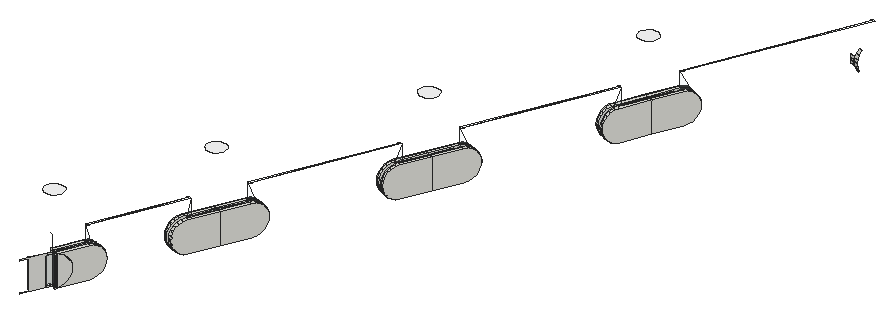
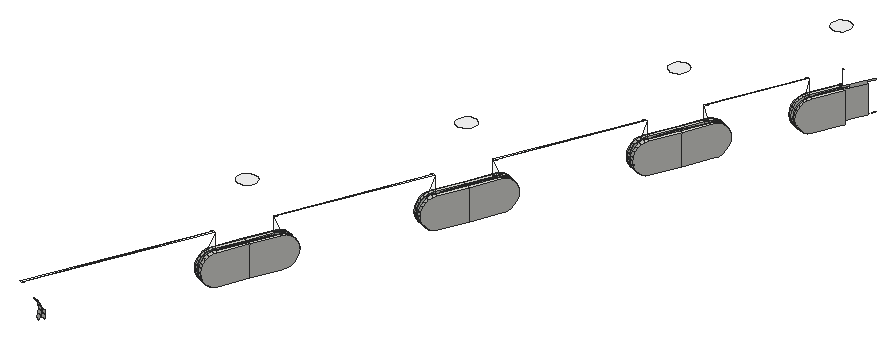
# SketchUp Ruby script. Lengths in inches.
U = 1.inch
M = Sketchup.active_model
def pt(a) = Geom::Point3d.new(a.map { |v| v * U })
def face(e, loops, mat)
  f = e.add_face(loops[0].map { |a| pt(a) })
  loops[1..].each { |l| e.add_face(l.map { |a| pt(a) }).erase! }
  f.material = f.back_material = mat if mat
  f
end
# faces: each face lists its corners as indices into pts; further lists are holes
def faces(e, pts, list, mat = nil) = list.each { |f| face(e, (f[0].is_a?(Array) ? f : [f]).map { |l| l.map { |i| pts[i] } }, mat) }
# xy, xz, yz: faces in a plane at the given z, y or x. An outline is a flat list of corners, or four numbers for a rectangle; further outlines are holes
def ring(l) = l.size == 4 ? [[l[0], l[1]], [l[2], l[1]], [l[2], l[3]], [l[0], l[3]]] : l.each_slice(2).to_a
def flat(e, list, mat, &to3) = list.each { |f| face(e, (f[0].is_a?(Array) ? f : [f]).map { |l| ring(l).map { |u, v| to3.(u, v) } }, mat) }
def xy(e, z, list, mat = nil) = flat(e, list, mat) { |x, y| [x, y, z] }
def xz(e, y, list, mat = nil) = flat(e, list, mat) { |x, z| [x, y, z] }
def yz(e, x, list, mat = nil) = flat(e, list, mat) { |y, z| [x, y, z] }
def lines(e, pts, list) = list.each { |a, b| e.add_line(pt(pts[a]), pt(pts[b])) }
# prism: a flat outline (further loops are holes) pulled along v
def prism(e, loops, v, mat = nil)
  f = face(e, loops, mat); d = Geom::Vector3d.new(v.map { |x| x * U })
  f.pushpull(f.normal.samedirection?(d) ? d.length : -d.length)
end
def box(e, o, s, mat = nil) = prism(e, [[o, [o[0] + s[0], o[1], o[2]], [o[0] + s[0], o[1] + s[1], o[2]], [o[0], o[1] + s[1], o[2]]]], [0, 0, s[2]], mat)
def at(x, y, z, deg = 0) = Geom::Transformation.translation(pt([x, y, z])) * Geom::Transformation.rotation(ORIGIN, Z_AXIS, deg.degrees)
def axes(o, x, y, z) = Geom::Transformation.new([*x, 0, *y, 0, *z, 0, *pt(o).to_a, 1])
def part(name) = M.definitions.add(name)
# library, detail: a bought-in or finely detailed component or shape, given as its bounding box
def library(name, o, s) = part(name).tap { |d| box(d.entities, o, s) }
def detail(e, o, s) = box(e.add_group.entities, o, s)
def put(e, d, t, mat = nil) = e.add_instance(d, t).tap { |i| i.material = mat if mat }
def group(e, t, mat = nil) = e.add_group.tap { |g| g.transformation = t; g.material = mat if mat }.entities
root = M.entities
M.materials.add("Glass_Safety_01").color = [204, 235, 244]
M.materials["Glass_Safety_01"].alpha = 0.1
M.materials.add("[Color_000]").color = [255, 255, 255]
xy(root,351.283,[[844.286,537.43,844.039,537.551,844.043,537.56,844.044,537.562,844.108,537.692,844.355,537.571],[844.362,537.586,844.11,537.696,844.896,539.501,845.148,539.391],[843.931,537.779,843.684,537.9,844.463,539.689,844.715,539.579],[847.571,544.953,847.318,545.063,847.473,545.418,848.104,546.868,848.357,546.758],[847.138,545.142,846.885,545.252,847.671,547.057,847.924,546.947,847.293,545.497],
  [848.357,546.758,848.104,546.868,848.89,548.673,849.143,548.563],[847.924,546.947,847.671,547.057,848.457,548.861,848.71,548.751],[852.79,556.936,852.537,557.046,852.656,557.318,853.323,558.851,853.576,558.741],[852.357,557.125,852.104,557.235,852.89,559.04,853.143,558.93,852.475,557.397],[853.576,558.741,853.323,558.851,854.109,560.656,854.362,560.546],
  [853.143,558.93,852.89,559.04,853.676,560.845,853.929,560.735],[858.192,569.34,857.939,569.45,858.054,569.713,858.726,571.255,858.978,571.145],[857.759,569.529,857.506,569.639,858.292,571.443,858.545,571.333,857.873,569.791],[858.978,571.145,858.726,571.255,859.512,573.06,859.764,572.949],[858.545,571.333,858.292,571.443,859.078,573.248,859.331,573.138]])
xy(root,351.362,[[843.866,537.198,843.689,537.285,843.862,537.638,843.867,537.648,843.929,537.775,844.019,537.735,844.108,537.692,844.044,537.562,844.043,537.56,844.039,537.551],[844.11,537.696,844.019,537.735,843.931,537.779,844.558,539.218,844.738,539.14],[844.019,537.735,843.929,537.775,843.931,537.779],[847.476,545.424,847.295,545.503,847.924,546.947,848.104,546.868],[848.104,546.868,847.924,546.947,848.553,548.39,848.733,548.312],
  [852.695,557.407,852.514,557.486,853.143,558.93,853.323,558.851],[853.323,558.851,853.143,558.93,853.772,560.374,853.952,560.295],[858.097,569.811,857.916,569.89,858.545,571.333,858.726,571.255],[858.726,571.255,858.545,571.333,859.174,572.777,859.354,572.699]],"Glass_Safety_01")
xy(root,353.33,[[844.11,537.696,844.738,539.14,844.558,539.218,843.931,537.779,844.019,537.735],[844.019,537.735,843.931,537.779,843.929,537.775],[847.476,545.424,848.104,546.868,847.924,546.947,847.295,545.503],[848.104,546.868,848.733,548.312,848.553,548.39,847.924,546.947],[852.695,557.407,853.323,558.851,853.143,558.93,852.514,557.486],
  [853.323,558.851,853.952,560.295,853.772,560.374,853.143,558.93],[858.097,569.811,858.726,571.255,858.545,571.333,857.916,569.89],[858.726,571.255,859.354,572.699,859.174,572.777,858.545,571.333]],"Glass_Safety_01")
xy(root,353.409,[[844.286,537.43,844.355,537.571,844.108,537.692,844.044,537.561,844.039,537.551],[844.362,537.586,845.148,539.391,844.896,539.501,844.11,537.696],[843.931,537.779,844.715,539.579,844.463,539.689,843.684,537.9],[847.571,544.953,848.357,546.758,848.104,546.868,847.473,545.418,847.347,545.13,847.318,545.063],[847.138,545.142,847.293,545.497,847.924,546.947,847.671,547.057,846.885,545.252],
  [848.357,546.758,849.143,548.563,848.89,548.673,848.104,546.868],[847.924,546.947,848.71,548.751,848.457,548.861,847.671,547.057],[852.79,556.936,853.576,558.741,853.323,558.851,852.656,557.318,852.537,557.046],[852.357,557.125,852.475,557.397,853.143,558.93,852.89,559.04,852.104,557.235],[853.576,558.741,854.362,560.546,854.109,560.656,853.323,558.851],
  [853.143,558.93,853.929,560.735,853.676,560.845,852.89,559.04],[858.192,569.34,858.978,571.145,858.726,571.255,858.054,569.713,857.939,569.45],[857.759,569.529,857.873,569.791,858.545,571.333,858.292,571.443,857.506,569.639],[858.978,571.145,859.764,572.949,859.512,573.06,858.726,571.255],[858.545,571.333,859.331,573.138,859.078,573.248,858.292,571.443]])
xy(root,354.511,[[844.039,537.551,844.044,537.562,843.867,537.648],[844.896,539.501,847.293,545.497,844.715,539.579],[844.896,539.501,847.473,545.418,847.293,545.497],[848.89,548.673,852.475,557.397,848.71,548.751],[848.89,548.673,852.656,557.318,852.475,557.397],
  [854.109,560.656,857.873,569.791,853.929,560.735],[854.109,560.656,858.054,569.713,857.873,569.791],[859.512,573.06,864.112,584.115,859.331,573.138],[859.512,573.06,864.292,584.037,864.112,584.115]],"Glass_Safety_01")
xy(root,357.267,[[844.064,537.107,844.226,537.14,844.373,537.214,844.496,537.323,844.586,537.46,844.638,537.616,844.648,537.78,844.615,537.941,844.541,538.088,844.432,538.211,844.295,538.302,844.139,538.354,843.974,538.364,843.813,538.331,843.666,538.257,843.543,538.148,843.453,538.01,843.401,537.854,843.391,537.69,843.424,537.529,843.498,537.382,843.607,537.259,843.744,537.169,843.9,537.117],[848.059,546.279,848.22,546.312,848.367,546.386,848.49,546.495,848.581,546.632,848.633,546.788,848.642,546.952,848.609,547.113,848.536,547.26,848.427,547.383,848.289,547.474,848.133,547.526,847.969,547.536,847.808,547.503,847.661,547.429,847.538,547.32,847.447,547.182,847.396,547.026,847.386,546.862,847.419,546.701,847.492,546.554,847.602,546.431,847.739,546.341,847.895,546.289],[853.278,558.262,853.439,558.295,853.586,558.369,853.709,558.478,853.8,558.615,853.852,558.771,853.861,558.936,853.828,559.097,853.755,559.244,853.646,559.367,853.508,559.457,853.352,559.509,853.188,559.519,853.027,559.486,852.88,559.412,852.757,559.303,852.667,559.166,852.615,559.01,852.605,558.846,852.638,558.684,852.712,558.537,852.821,558.414,852.958,558.324,853.114,558.272],[858.68,570.666,858.841,570.699,858.988,570.772,859.111,570.882,859.202,571.019,859.254,571.175,859.264,571.339,859.231,571.5,859.157,571.647,859.048,571.77,858.91,571.861,858.754,571.913,858.59,571.922,858.429,571.889,858.282,571.816,858.159,571.707,858.069,571.569,858.017,571.413,858.007,571.249,858.04,571.088,858.114,570.941,858.223,570.818,858.36,570.727,858.516,570.676]],"[Color_000]")
p = [[843.173,535.784,353.33],[843.173,535.784,353.388],[843.242,535.924,353.409],[844.039,537.551,353.409],[844.044,537.561,353.408],[844.108,537.692,353.388],
  [844.108,537.692,353.33],[844.044,537.561,353.33],[844.044,537.562,351.362],[844.108,537.692,351.362],[844.11,537.696,353.388],[844.16,537.799,353.373],
  [844.273,538.029,353.267],[844.37,538.226,353.098],[844.444,538.378,352.877],[844.491,538.474,352.621],[844.507,538.506,352.346],[844.491,538.474,352.071],
  [844.444,538.378,351.815],[844.37,538.226,351.594],[844.273,538.029,351.425],[844.16,537.799,351.319],[844.11,537.696,351.304],[844.108,537.692,351.304],
  [844.044,537.562,351.285],[844.043,537.56,351.284],[844.039,537.551,351.283],[843.242,535.924,351.283],[843.173,535.784,351.304],[843.173,535.784,351.362],
  [843.415,536.278,351.362],[843.415,536.278,353.33],[843.866,537.198,351.362],[844.039,537.551,351.362],[844.039,537.551,353.33],[843.866,537.198,353.33],
  [843.238,536.364,353.33],[843.238,536.364,351.362],[843.689,537.285,351.362],[843.862,537.638,351.362],[843.862,537.638,351.283],[843.863,537.64,351.283],
  [843.867,537.648,351.285],[843.929,537.775,351.303],[843.931,537.779,351.304],[843.983,537.885,351.319],[844.096,538.115,351.425],[844.193,538.313,351.594],
  [844.267,538.465,351.815],[844.314,538.56,352.071],[844.33,538.593,352.346],[844.314,538.56,352.621],[844.267,538.465,352.877],[844.193,538.313,353.098],
  [844.096,538.115,353.267],[843.983,537.885,353.373],[843.931,537.779,353.388],[843.929,537.775,353.389],[843.867,537.648,353.407],[843.862,537.638,353.409],
  [843.862,537.638,353.33],[843.689,537.285,353.33],[844.407,537.677,351.319],[844.362,537.586,351.306],[844.355,537.571,351.304],[844.286,537.43,351.283],
  [844.355,537.571,351.283],[844.043,537.56,351.362],[844.043,537.56,351.283],[844.044,537.562,351.283],[844.108,537.692,351.283],[844.108,537.692,353.409],
  [844.355,537.571,353.409],[844.355,537.571,353.388],[844.11,537.696,351.283],[844.362,537.586,351.283],[844.362,537.586,353.386],[844.362,537.586,353.409],
  [844.11,537.696,353.409],[844.11,537.696,353.33],[844.11,537.696,351.362],[844.407,537.677,353.373],[844.52,537.908,351.425],[844.617,538.105,351.594],
  [844.691,538.257,351.815],[844.738,538.352,352.071],[844.754,538.385,352.346],[844.738,538.352,352.621],[844.691,538.257,352.877],[844.617,538.105,353.098],
  [844.52,537.908,353.267],[845.148,539.391,353.409],[845.148,539.391,351.283],[845.258,539.643,351.319],[845.361,539.878,351.425],[845.448,540.08,351.594],
  [845.516,540.235,351.815],[845.558,540.332,352.071],[845.573,540.365,352.346],[845.558,540.332,352.621],[845.516,540.235,352.877],[845.448,540.08,353.098],
  [845.361,539.878,353.267],[845.258,539.643,353.373],[844.896,539.501,353.409],[845.006,539.753,353.373],[845.108,539.988,353.267],[845.196,540.19,353.098],
  [845.263,540.345,352.877],[845.306,540.442,352.621],[845.32,540.475,352.346],[845.306,540.442,352.071],[845.263,540.345,351.815],[845.196,540.19,351.594],
  [845.108,539.988,351.425],[845.006,539.753,351.319],[844.896,539.501,351.283],[843.931,537.779,353.409],[843.929,537.775,353.409],[843.929,537.775,353.33],
  [843.929,537.775,351.362],[843.929,537.775,351.283],[843.931,537.779,351.283],[844.715,539.579,351.283],[844.825,539.832,351.319],[844.927,540.067,351.425],
  [845.015,540.268,351.594],[845.039,540.323,351.671],[845.083,540.423,351.815],[845.125,540.521,352.071],[845.14,540.554,352.346],[845.125,540.521,352.621],
  [845.083,540.423,352.877],[845.015,540.268,353.098],[844.927,540.067,353.267],[844.848,539.883,353.349],[844.825,539.832,353.373],[844.715,539.579,353.409],
  [843.677,537.885,353.409],[843.68,537.892,353.409],[843.684,537.9,353.409],[844.463,539.689,353.409],[844.572,539.942,353.373],[844.675,540.177,353.267],
  [844.763,540.379,353.098],[844.83,540.533,352.877],[844.873,540.631,352.621],[844.887,540.664,352.346],[844.873,540.631,352.071],[844.83,540.533,351.815],
  [844.763,540.379,351.594],[844.675,540.177,351.425],[844.572,539.942,351.319],[844.463,539.689,351.283],[843.684,537.9,351.283],[843.68,537.892,351.283],
  [843.677,537.885,351.283],[843.676,537.885,351.301],[843.676,537.885,353.391],[848.357,546.758,353.409],[847.571,544.953,353.409],[847.461,544.701,353.373],
  [847.359,544.466,353.267],[847.271,544.264,353.098],[847.203,544.109,352.877],[847.161,544.012,352.621],[847.147,543.979,352.346],[847.161,544.012,352.071],
  [847.203,544.109,351.815],[847.271,544.264,351.594],[847.359,544.466,351.425],[847.461,544.701,351.319],[847.571,544.953,351.283],[848.357,546.758,351.283],
  [847.138,545.142,351.283],[847.293,545.497,351.283],[847.293,545.497,353.409],[847.138,545.142,353.409],[847.028,544.89,353.373],[846.926,544.655,353.267],
  [846.838,544.453,353.098],[846.77,544.298,352.877],[846.728,544.2,352.621],[846.713,544.167,352.346],[846.728,544.2,352.071],[846.77,544.298,351.815],
  [846.838,544.453,351.594],[846.926,544.655,351.425],[847.028,544.89,351.319],[846.885,545.252,353.409],[847.671,547.057,353.409],[847.671,547.057,351.283],
  [846.885,545.252,351.283],[846.775,545,351.319],[846.673,544.765,351.425],[846.585,544.563,351.594],[846.518,544.408,351.815],[846.475,544.311,352.071],
  [846.461,544.277,352.346],[846.475,544.311,352.621],[846.518,544.408,352.877],[846.585,544.563,353.098],[846.673,544.765,353.267],[846.775,545,353.373],
  [847.106,544.576,351.425],[847.12,544.607,351.411],[847.208,544.811,351.319],[847.347,545.13,353.409],[847.473,545.418,353.409],[847.473,545.418,351.283],
  [847.318,545.063,351.283],[848.104,546.868,351.283],[848.104,546.868,353.409],[848.104,546.868,353.33],[847.476,545.424,353.33],[847.476,545.424,351.362],
  [848.104,546.868,351.362],[847.924,546.947,353.409],[847.924,546.947,351.283],[847.924,546.947,351.362],[847.295,545.503,351.362],[847.295,545.503,353.33],
  [847.924,546.947,353.33],[849.143,548.563,353.409],[849.143,548.563,351.283],[849.253,548.815,351.319],[849.355,549.05,351.425],[849.443,549.252,351.594],
  [849.511,549.407,351.815],[849.553,549.504,352.071],[849.567,549.537,352.346],[849.553,549.504,352.621],[849.511,549.407,352.877],[849.443,549.252,353.098],
  [849.355,549.05,353.267],[849.253,548.815,353.373],[848.71,548.751,351.283],[848.71,548.751,353.409],[848.553,548.39,353.33],[848.553,548.39,351.362],
  [848.89,548.673,353.409],[848.89,548.673,351.283],[848.733,548.312,351.362],[848.733,548.312,353.33],[848.457,548.861,353.409],[848.567,549.114,353.373],
  [848.669,549.349,353.267],[848.757,549.551,353.098],[848.825,549.705,352.877],[848.867,549.803,352.621],[848.882,549.836,352.346],[848.867,549.803,352.071],
  [848.825,549.705,351.815],[848.757,549.551,351.594],[848.669,549.349,351.425],[848.567,549.114,351.319],[848.457,548.861,351.283],[849,548.925,351.319],
  [849.103,549.16,351.425],[849.191,549.362,351.594],[849.258,549.517,351.815],[849.3,549.614,352.071],[849.315,549.647,352.346],[849.3,549.614,352.621],
  [849.258,549.517,352.877],[849.191,549.362,353.098],[849.103,549.16,353.267],[849,548.925,353.373],[848.82,549.004,351.319],[848.922,549.239,351.425],
  [849.01,549.44,351.594],[849.077,549.595,351.815],[849.118,549.689,352.06],[848.916,549.225,353.273],[848.82,549.004,353.373],[853.576,558.741,353.409],
  [852.79,556.936,353.409],[852.68,556.684,353.373],[852.578,556.449,353.267],[852.49,556.247,353.098],[852.422,556.092,352.877],[852.38,555.995,352.621],
  [852.366,555.962,352.346],[852.38,555.995,352.071],[852.422,556.092,351.815],[852.49,556.247,351.594],[852.578,556.449,351.425],[852.68,556.684,351.319],
  [852.79,556.936,351.283],[853.576,558.741,351.283],[852.357,557.125,351.283],[852.475,557.397,351.283],[852.475,557.397,353.409],[852.357,557.125,353.409],
  [852.247,556.873,353.373],[852.145,556.638,353.267],[852.057,556.436,353.098],[851.989,556.281,352.877],[851.947,556.184,352.621],[851.932,556.151,352.346],
  [851.947,556.184,352.071],[851.989,556.281,351.815],[852.057,556.436,351.594],[852.145,556.638,351.425],[852.247,556.873,351.319],[852.104,557.235,353.409],
  [852.89,559.04,353.409],[852.89,559.04,351.283],[852.104,557.235,351.283],[851.994,556.983,351.319],[851.892,556.748,351.425],[851.804,556.546,351.594],
  [851.737,556.391,351.815],[851.694,556.294,352.071],[851.68,556.261,352.346],[851.694,556.294,352.621],[851.737,556.391,352.877],[851.804,556.546,353.098],
  [851.892,556.748,353.267],[851.994,556.983,353.373],[852.656,557.318,353.409],[852.656,557.318,351.283],[852.537,557.046,351.283],[852.428,556.794,351.319],
  [852.325,556.559,351.425],[852.237,556.357,351.594],[852.194,556.257,351.736],[852.468,556.888,353.386],[852.537,557.046,353.409],[853.323,558.851,351.283],
  [853.323,558.851,353.409],[853.323,558.851,353.33],[852.695,557.407,353.33],[852.695,557.407,351.362],[853.323,558.851,351.362],[853.143,558.93,353.409],
  [853.143,558.93,351.283],[853.143,558.93,351.362],[852.514,557.486,351.362],[852.514,557.486,353.33],[853.143,558.93,353.33],[854.362,560.546,353.409],
  [854.362,560.546,351.283],[854.472,560.798,351.319],[854.574,561.033,351.425],[854.662,561.235,351.594],[854.73,561.39,351.815],[854.772,561.487,352.071],
  [854.787,561.521,352.346],[854.772,561.487,352.621],[854.73,561.39,352.877],[854.662,561.235,353.098],[854.574,561.033,353.267],[854.472,560.798,353.373],
  [853.929,560.735,351.283],[853.929,560.735,353.409],[853.772,560.374,353.33],[853.772,560.374,351.362],[854.109,560.656,353.409],[854.109,560.656,351.283],
  [853.952,560.295,351.362],[853.952,560.295,353.33],[853.676,560.845,353.409],[853.786,561.097,353.373],[853.889,561.332,353.267],[853.976,561.534,353.098],
  [854.044,561.689,352.877],[854.086,561.786,352.621],[854.101,561.819,352.346],[854.086,561.786,352.071],[854.044,561.689,351.815],[853.976,561.534,351.594],
  [853.889,561.332,351.425],[853.786,561.097,351.319],[853.676,560.845,351.283],[854.219,560.908,351.319],[854.039,560.987,351.319],[854.141,561.222,351.425],
  [854.229,561.424,351.594],[854.297,561.579,351.815],[854.339,561.676,352.071],[854.343,561.684,352.14],[854.149,561.239,353.252],[854.141,561.222,353.267],
  [854.039,560.987,353.373],[854.322,561.143,351.425],[854.41,561.345,351.594],[854.477,561.5,351.815],[854.519,561.597,352.071],[854.534,561.631,352.346],
  [854.519,561.597,352.621],[854.477,561.5,352.877],[854.41,561.345,353.098],[854.322,561.143,353.267],[854.219,560.908,353.373],[858.978,571.145,353.409],
  [858.192,569.34,353.409],[858.082,569.088,353.373],[857.98,568.853,353.267],[857.892,568.651,353.098],[857.825,568.496,352.877],[857.782,568.399,352.621],
  [857.768,568.365,352.346],[857.782,568.399,352.071],[857.825,568.496,351.815],[857.892,568.651,351.594],[857.98,568.853,351.425],[858.082,569.088,351.319],
  [858.192,569.34,351.283],[858.978,571.145,351.283],[857.759,569.529,351.283],[857.873,569.791,351.283],[857.873,569.791,353.409],[857.759,569.529,353.409],
  [857.649,569.276,353.373],[857.547,569.041,353.267],[857.459,568.839,353.098],[857.391,568.685,352.877],[857.349,568.587,352.621],[857.335,568.554,352.346],
  [857.349,568.587,352.071],[857.391,568.685,351.815],[857.459,568.839,351.594],[857.547,569.041,351.425],[857.649,569.276,351.319],[858.054,569.713,353.409],
  [858.054,569.713,351.283],[857.939,569.45,351.283],[857.83,569.198,351.319],[857.727,568.963,351.425],[857.639,568.761,351.594],[857.579,568.623,351.79],
  [857.857,569.26,353.382],[857.939,569.45,353.409],[857.506,569.639,353.409],[858.292,571.443,353.409],[858.292,571.443,351.283],[857.506,569.639,351.283],
  [857.396,569.386,351.319],[857.294,569.151,351.425],[857.206,568.95,351.594],[857.139,568.795,351.815],[857.096,568.697,352.071],[857.082,568.664,352.346],
  [857.096,568.697,352.621],[857.139,568.795,352.877],[857.206,568.95,353.098],[857.294,569.151,353.267],[857.396,569.386,353.373],[858.726,571.255,351.283],
  [858.726,571.255,353.409],[858.726,571.255,353.33],[858.097,569.811,353.33],[858.097,569.811,351.362],[858.726,571.255,351.362],[858.545,571.333,353.409],
  [858.545,571.333,351.283],[858.545,571.333,351.362],[857.916,569.89,351.362],[857.916,569.89,353.33],[858.545,571.333,353.33],[859.764,572.949,353.409],
  [859.764,572.949,351.283],[859.874,573.202,351.319],[859.976,573.437,351.425],[860.064,573.639,351.594],[860.132,573.793,351.815],[860.174,573.891,352.071],
  [860.189,573.924,352.346],[860.174,573.891,352.621],[860.132,573.793,352.877],[860.064,573.639,353.098],[859.976,573.437,353.267],[859.874,573.202,353.373],
  [859.331,573.138,351.283],[859.331,573.138,353.409],[859.174,572.777,353.33],[859.174,572.777,351.362],[859.512,573.06,353.409],[859.512,573.06,351.283],
  [859.354,572.699,351.362],[859.354,572.699,353.33],[859.078,573.248,353.409],[859.188,573.5,353.373],[859.291,573.735,353.267],[859.379,573.9375,353.098],
  [859.446,574.092,352.877],[859.488,574.19,352.621],[859.503,574.223,352.346],[859.488,574.19,352.071],[859.446,574.092,351.815],[859.379,573.9375,351.594],
  [859.291,573.735,351.425],[859.188,573.5,351.319],[859.078,573.248,351.283],[859.621,573.312,351.319],[859.441,573.39,351.319],[859.543,573.625,351.425],
  [859.631,573.827,351.594],[859.699,573.982,351.815],[859.741,574.08,352.071],[859.756,574.113,352.346],[859.745,574.087,352.556],[859.629,573.822,353.102],
  [859.543,573.625,353.267],[859.441,573.39,353.373],[859.724,573.547,351.425],[859.812,573.749,351.594],[859.879,573.904,351.815],[859.922,574.001,352.071],
  [859.936,574.034,352.346],[859.922,574.001,352.621],[859.879,573.904,352.877],[859.812,573.749,353.098],[859.724,573.547,353.267],[859.621,573.312,353.373],
  [844.019,537.735,351.362],[844.019,537.735,353.33],[843.931,537.779,353.33],[843.931,537.779,351.362],[844.738,539.14,353.33],[844.738,539.14,351.362],
  [844.558,539.218,351.362],[844.558,539.218,353.33],[843.849,538.237,351.425],[843.945,538.434,351.594],[847.018,544.374,351.594],[846.951,544.219,351.815],
  [846.908,544.122,352.071],[846.894,544.089,352.346],[846.908,544.122,352.621],[846.951,544.219,352.877],[847.018,544.374,353.098],[847.106,544.576,353.267],
  [847.208,544.811,353.373],[847.318,545.063,353.409],[844.02,538.586,351.815],[852.17,556.202,351.815],[857.572,568.606,351.815],[852.127,556.105,352.071],
  [852.113,556.072,352.346],[852.127,556.105,352.621],[852.17,556.202,352.877],[852.237,556.357,353.098],[852.325,556.559,353.267],[852.428,556.794,353.373],
  [844.066,538.681,352.071],[849.12,549.693,352.071],[857.53,568.509,352.071],[857.515,568.475,352.346],[857.53,568.509,352.621],[857.572,568.606,352.877],
  [857.639,568.761,353.098],[857.727,568.963,353.267],[857.83,569.198,353.373],[863.784,582.869,352.071],[863.826,582.966,351.815],[864.079,582.856,351.815],
  [864.036,582.759,352.071],[844.082,538.714,352.346],[848.922,549.239,353.267],[849.01,549.44,353.098],[849.077,549.595,352.877],[849.12,549.693,352.621],
  [849.134,549.726,352.346],[854.229,561.424,353.098],[854.297,561.579,352.877],[854.339,561.676,352.621],[854.353,561.709,352.346],[863.769,582.835,352.346],
  [863.782,582.865,352.098],[864.022,582.725,352.346],[863.603,582.947,352.071],[863.589,582.914,352.346],[863.336,583.024,352.346],[863.351,583.057,352.071],
  [844.066,538.681,352.621],[859.741,574.08,352.621],[863.784,582.869,352.621],[864.036,582.759,352.621],[863.603,582.947,352.621],[863.351,583.057,352.621],
  [844.02,538.586,352.877],[859.631,573.827,353.098],[859.699,573.982,352.877],[863.826,582.966,352.877],[864.079,582.856,352.877],[843.945,538.434,353.098],
  [863.894,583.121,353.098],[864.146,583.011,353.098],[843.849,538.237,353.267],[859.331,573.138,354.511],[844.715,539.579,354.511],[848.71,548.751,354.511],
  [853.929,560.735,354.511],[844.286,537.43,353.409],[844.039,537.551,354.511],[844.044,537.561,353.409],[844.044,537.562,354.511],[847.473,545.418,354.511],
  [852.656,557.318,354.511],[858.054,569.713,354.511]]
faces(root,p,[[[0,1,2,3,4,5,6,7,8,9,6,5,10,11,12,13,14,15,16,17,18,19,20,21,22,23,24,25,26,27,28,29,30,31],[32,33,34,35]],[36,37,38,39,40,41,42,43,44,45,46,47,48,49,50,51,52,53,54,55,56,57,58,59,60,61],[22,21,62,63,64,65,26,25,24,23],[66,64,65],[70,69,24,23],[70,23,9,6,5,71,72,73,64,66],[22,74,75,63,76,77,78,10,79,80],[64,63,76,73],
  [81,76,63,62,82,83,84,85,86,87,88,89,90],[91,77,76,63,75,92,93,94,95,96,97,98,99,100,101,102,103],[78,104,105,106,107,108,109,110,111,112,113,114,115,116,74,22,80,79,10],[21,20,82,62],[117,118,57,119,120,43,121,122,123,124,125,126,127,128,129,130,131,132,133,134,135,136,137],[138,139,140,141,142,143,144,145,146,147,148,149,150,151,152,153,154,155,156,157,158],[116,115,93,92],[124,123,153,152],
  [115,114,94,93],[125,124,152,151],[159,160,161,162,163,164,165,166,167,168,169,170,171,172,173],[174,175,176,177,178,179,180,181,182,183,184,185,186,187,188],[189,190,191,192,193,194,195,196,197,198,199,200,201,202,203],[204,205,206,171,170],[207,208,209,210,206,205],[188,187,194,193],
  [206,210,172,171],[174,188,193,192],[211,209,208,212,213,214,215,216],[217,176,175,218,219,220,221,222],[211,216,213,212,159,173],[223,159,173,224,225,226,227,228,229,230,231,232,233,234,235],[219,218,191,190,217,222],[218,236,237,217,222,238,239,219],
  [212,240,241,211,216,242,243,213],[190,244,245,246,247,248,249,250,251,252,253,254,255,256,191],[241,257,225,224],[268,236,256,255],[257,258,226,225],[269,268,255,254],[275,276,277,278,279,280,281,282,283,284,285,286,287,288,289],[290,291,292,293,294,295,296,297,298,299,300,301,302,303,304],
  [305,306,307,308,309,310,311,312,313,314,315,316,317,318,319],[324,323,287,286],[304,303,310,309],[323,322,288,287],[290,304,309,308],[329,321,320,330,331,332,333,334],[335,292,291,336,337,338,339,340],[329,334,331,330,275,289],
  [341,275,289,342,343,344,345,346,347,348,349,350,351,352,353],[337,336,307,306,335,340],[336,354,355,335,340,356,357,337],[330,358,359,329,334,360,361,331],[306,362,363,364,365,366,367,368,369,370,371,372,373,374,307],[359,375,343,342],[376,354,374,373],[375,385,344,343],
  [377,376,373,372],[395,396,397,398,399,400,401,402,403,404,405,406,407,408,409],[410,411,412,413,414,415,416,417,418,419,420,421,422,423,424],[434,435,436,437,438,439,440,441,442,443,444,445,446,447,448],[429,428,407,406],[424,423,439,438],[428,427,408,407],[410,424,438,437],
  [449,426,425,450,451,452,453,454],[455,412,411,456,457,458,459,460],[449,454,451,450,395,409],[461,395,409,462,463,464,465,466,467,468,469,470,471,472,473],[457,456,436,435,455,460],[456,474,475,455,460,476,477,457],[450,478,479,449,454,480,481,451],[435,482,483,484,485,486,487,488,489,490,491,492,493,494,436],
  [479,495,463,462],[496,474,494,493],[495,506,464,463],[497,496,493,492],[20,19,83,82],[47,46,524,525],[114,113,95,94],[126,125,151,150],
  [526,204,170,169],[187,186,195,194],[258,259,227,226],[270,269,254,253],[325,324,286,285],[303,302,311,310],[385,386,345,344],[378,377,372,371],
  [430,429,406,405],[423,422,440,439],[506,507,465,464],[498,497,492,491],[19,18,84,83],[48,47,525,536],[113,112,96,95],[128,127,126,150,149],
  [527,526,169,168],[186,185,196,195],[259,260,228,227],[271,270,253,252],[537,326,325,285,284],[302,301,312,311],[386,387,346,345],[379,378,371,370],
  [538,431,430,405,404],[422,421,441,440],[507,508,466,465],[499,498,491,490],[326,537,539,540,541,542,543,544,545,327],[18,17,85,84],[49,48,536,546],[112,111,97,96],
  [129,128,149,148],[528,527,168,167],[185,184,197,196],[260,261,229,228],[547,272,271,252,251],[539,537,284,283],[301,300,313,312],[387,388,347,346],
  [380,379,370,369],[548,538,404,403],[431,538,548,549,550,551,552,553,554,432],[421,420,442,441],[508,509,467,466],[500,499,490,489],[555,556,557,558],[17,16,86,85],
  [50,49,546,559],[111,110,98,97],[130,129,148,147],[529,528,167,166],[184,183,198,197],[261,262,230,229],[564,547,251,250],[540,539,283,282],
  [300,299,314,313],[388,389,348,347],[568,381,380,369,368],[549,548,403,402],[420,419,443,442],[509,510,468,467],[501,500,489,488],[569,570,555,558,571],
  [572,573,574,575],[16,15,87,86],[51,50,559,576],[110,109,99,98],[131,130,147,146],[530,529,166,165],[183,182,199,198],[262,263,231,230],
  [563,564,250,249],[541,540,282,281],[299,298,315,314],[389,390,349,348],[567,568,368,367],[550,549,402,401],[419,418,444,443],[510,511,469,468],
  [577,502,501,488,487],[578,569,571,579],[573,580,581,574],[15,14,88,87],[52,51,576,582],[109,108,100,99],[132,131,146,145],[531,530,165,164],
  [182,181,200,199],[263,264,232,231],[562,563,249,248],[542,541,281,280],[298,297,316,315],[390,391,350,349],[566,567,367,366],[551,550,401,400],
  [418,417,445,444],[511,512,470,469],[584,577,487,486],[585,578,579,586],[14,13,89,88],[53,52,582,587],[108,107,101,100],[133,132,145,144],
  [532,531,164,163],[181,180,201,200],[264,265,233,232],[561,562,248,247],[543,542,280,279],[297,296,317,316],[391,392,351,350],[565,566,366,365],
  [552,551,400,399],[417,416,446,445],[512,513,471,470],[583,584,486,485],[588,585,586,589],[13,12,90,89],[54,53,587,590],[107,106,102,101],
  [134,133,144,143],[533,532,163,162],[180,179,202,201],[265,266,234,233],[560,561,247,246],[544,543,279,278],[296,295,318,317],[392,393,352,351],
  [383,382,565,365,364],[553,552,399,398],[416,415,447,446],[513,514,472,471],[504,503,583,485,484],[12,11,81,90],[106,105,103,102],[136,135,134,143,142],
  [534,533,162,161],[179,178,203,202],[266,267,235,234],[274,273,560,246,245],[545,544,278,277],[295,294,319,318],[393,394,353,352],[384,383,364,363],
  [554,553,398,397],[415,414,448,447],[514,515,473,472],[505,504,484,483],[4,3,595,73,76,81,11,10,5],[72,595,73],[5,4,597,71],[105,104,91,103],
  [137,136,142,141],[535,534,161,160],[178,177,189,203],[267,240,223,235],[237,274,245,244],[328,327,545,277,276],[294,293,305,319],[394,358,341,353],
  [355,384,363,362],[433,432,554,397,396],[414,413,434,448],[515,478,461,473],[475,505,483,482]])
faces(root,p,[[26,33,67,25,68],[69,24,25,68],[67,25,24,8],[104,116,115,114,113,112,111,110,109,108,107,106,105],[123,137,136,135,127,126,125,124],[240,241,257,258,259,260,261,262,263,264,265,266,267],[237,236,268,269,270,271,272,273,274],[320,321,322,323,324,325,326,327,328],
  [355,354,376,377,378,379,380,381,382,383,384],[358,359,375,385,386,387,388,389,390,391,392,393,394],[425,426,427,428,429,430,431,432,433],[475,474,496,497,498,499,500,501,502,503,504,505],[478,479,495,506,507,508,509,510,511,512,513,514,515],[33,32,35,34],[33,34,7,67],[34,7,8,67,33],
  [67,7,8],[7,6,9,8],[516,517,119,120],[518,517,516,519],[9,516,517,6],[517,516,80,79],[520,79,80,521],[522,519,518,523],
  [521,522,523,520],[207,205,204,526,527,528,529,530,531,532,533,534,535],[221,220,215,214],[214,213,216,215],[222,221,220,219],[222,213,216,219],[238,222,219,239],[213,243,242,216],
  [243,242,239,238],[339,338,333,332],[332,331,334,333],[340,339,338,337],[340,331,334,337],[356,340,337,357],[331,361,360,334],[361,360,357,356],
  [459,458,453,452],[452,451,454,453],[460,459,458,457],[460,451,454,457],[476,460,457,477],[451,481,480,454],[481,480,477,476],[127,135,134,133,132,131,130,129,128],
  [272,273,560,561,562,563,564,547],[381,382,565,566,567,568],[502,503,583,584,577],[591,503,504,505,475],[4,7,34,3],[592,135,136,137],[593,273,274,237],[594,382,383,384,355],
  [596,3,597,598],[599,207,208],[600,327,328,320],[601,432,433,425]],"Glass_Safety_01")
